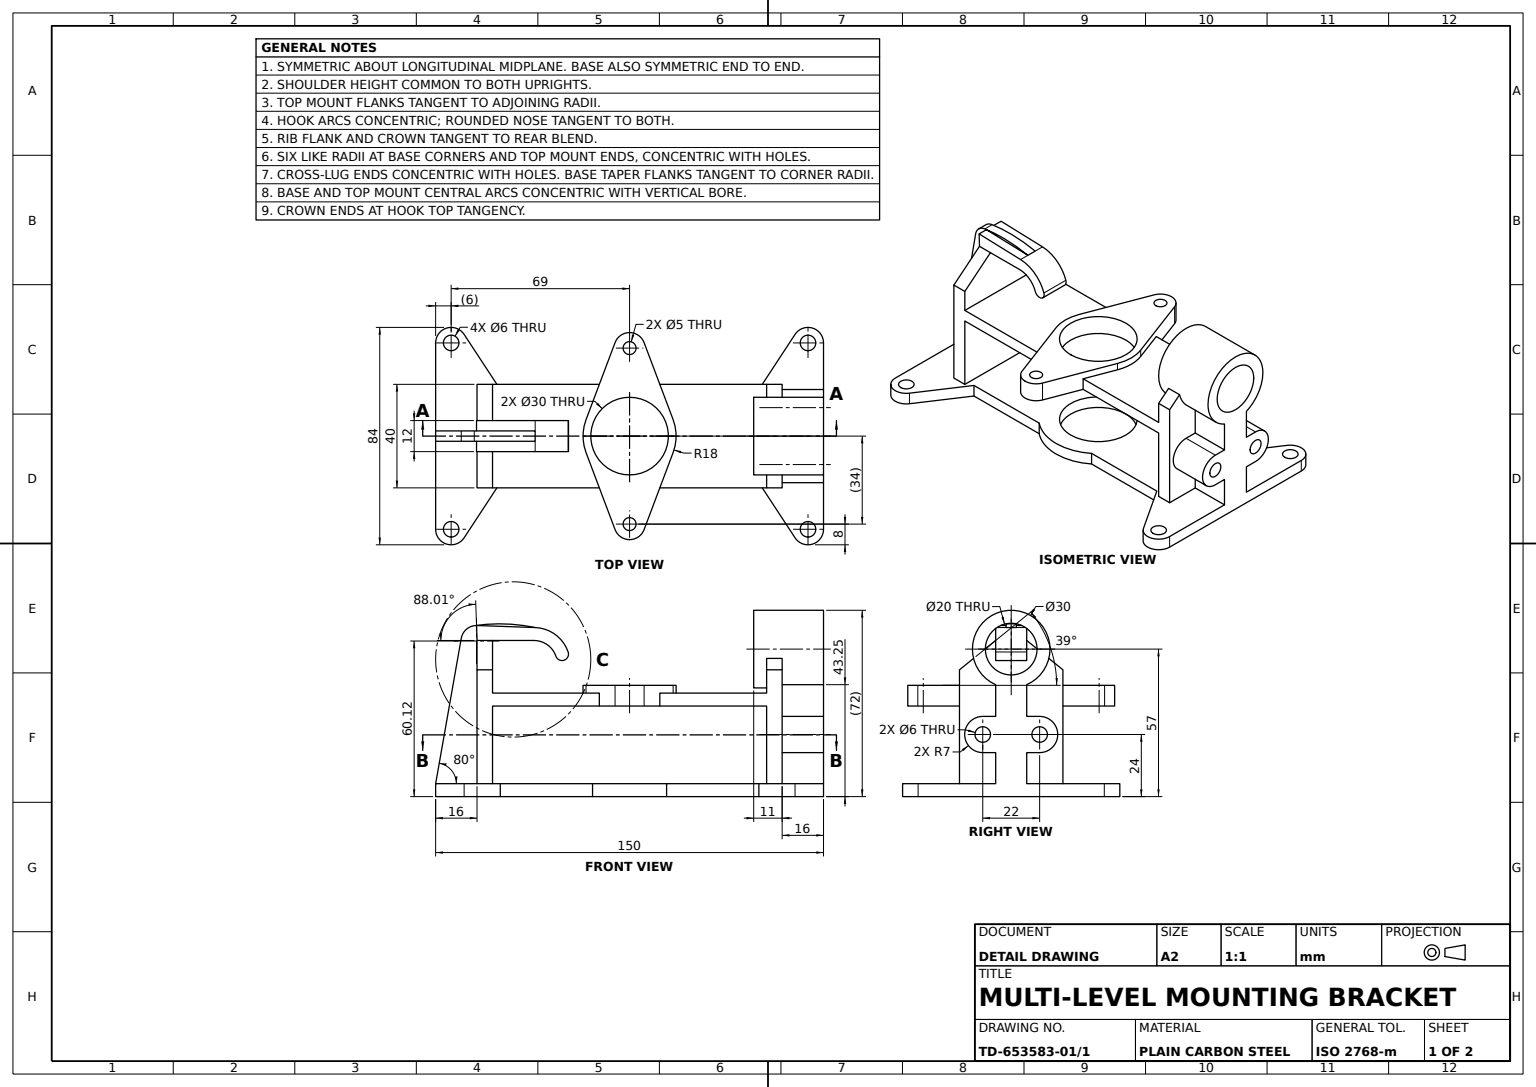
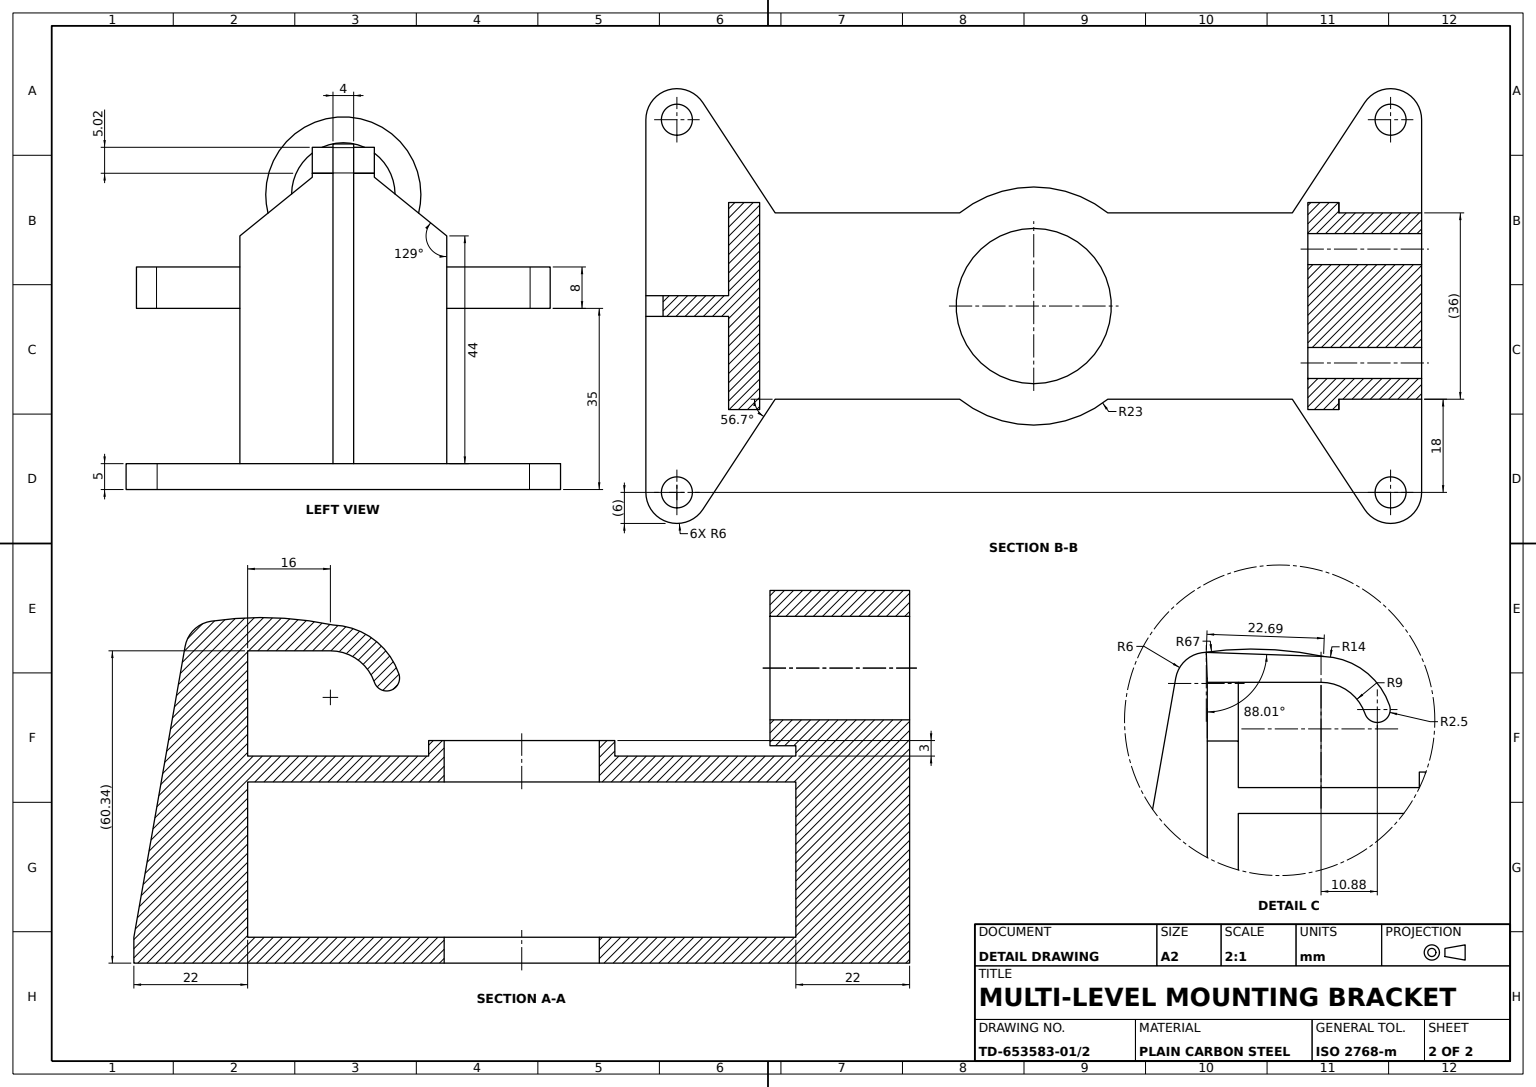
solid
v1 (-53,49,-20)
v2 (-53,40,-20)
e1 v1 v2 LINE
v3 (-53,53.403279,-14.562404)
e2 v1 v3 LINE
v4 (-53,53.403279,14.562404)
e3 v3 v4 CIRCLE(AX(P(-53,57,0),D(-1,0,0),D(0,0,1)),15)
v5 (-53,49,20)
e4 v5 v4 LINE
v6 (-53,40,20)
e5 v5 v6 LINE
e6 v6 v2 LINE
face PLANE(AX(P(-53,49,-20),D(-1,0,0),D(0,0,1))) rev [-e1 e2 e3 -e4 e5 e6]
v7 (0,43,36.5)
v8 (0,43,31.5)
e7 v7 v8 CIRCLE(AX(P(0,43,34),D(0,1,0),D(0,0,1)),2.5)
v9 (0,35,31.5)
e8 v8 v9 LINE
v10 (0,35,36.5)
e9 v10 v9 CIRCLE(AX(P(0,35,34),D(0,1,0),D(0,0,1)),2.5)
e10 v7 v10 LINE
face CYL(AX(P(0,43,34),D(0,-1,0),D(0,0,-1)),2.5) rev [e7 e8 -e9 -e10]
v11 (69,0,33)
v12 (69,0,39)
e11 v11 v12 CIRCLE(AX(P(69,0,36),D(0,1,0),D(0,0,1)),3)
v13 (69,5,33)
e12 v13 v11 LINE
v14 (69,5,39)
e13 v13 v14 CIRCLE(AX(P(69,5,36),D(0,1,0),D(0,0,1)),3)
e14 v14 v12 LINE
face CYL(AX(P(69,5,36),D(0,-1,0),D(0,0,-1)),3) rev [-e11 -e12 e13 e14]
v15 (63.984888,0,39.293729)
v16 (75,0,36)
e15 v15 v16 CIRCLE(AX(P(69,0,36),D(0,1,0),D(0,0,1)),6)
v17 (75,5,36)
e16 v17 v16 LINE
v18 (63.984888,5,39.293729)
e17 v18 v17 CIRCLE(AX(P(69,5,36),D(0,1,0),D(0,0,1)),6)
e18 v18 v15 LINE
face CYL(AX(P(69,5,36),D(0,-1,0),D(0,0,-1)),6) [e15 -e16 -e17 e18]
v19 (59.014781,61.103283,-6)
v20 (59,61.102768,-6)
e19 v19 v20 LINE
v21 (59.014781,61.103283,-2)
e20 v21 v19 LINE
v22 (59,61.102768,-2)
e21 v21 v22 LINE
e22 v20 v22 LINE
face PLANE(AX(P(-2.052934,58.977594,6),D(0.03478765,-0.999394727,0),D(0.999394727,0.03478765,0))) [-e19 -e20 e21 -e22]
v23 (-75,5,-6)
v24 (-75,17,-6)
e23 v23 v24 LINE
v25 (-59,17,-6)
e24 v24 v25 LINE
v26 (-59,5,-6)
e25 v25 v26 LINE
e26 v23 v26 LINE
face PLANE(AX(P(-153,43.252273,-6),D(0,0,1),D(1,0,0))) rev [e23 e24 e25 -e26]
v27 (-5.613873,35,36.117647)
v28 (5.613873,35,36.117647)
e27 v27 v28 CIRCLE(AX(P(0,35,34),D(0,1,0),D(0,0,1)),6)
v29 (5.613873,43,36.117647)
e28 v29 v28 LINE
v30 (-5.613873,43,36.117647)
e29 v30 v29 CIRCLE(AX(P(0,43,34),D(0,1,0),D(0,0,1)),6)
e30 v30 v27 LINE
face CYL(AX(P(0,43,34),D(0,-1,0),D(0,0,-1)),6) [e27 -e28 -e29 e30]
v31 (11.69372,35,-20)
v32 (5.613873,35,-36.117647)
e31 v31 v32 LINE
v33 (53,35,-20)
e32 v31 v33 LINE
v34 (53,35,20)
e33 v33 v34 LINE
v35 (11.69372,35,20)
e34 v35 v34 LINE
e35 v35 v28 LINE
v36 (-11.69372,35,20)
e36 v36 v27 LINE
v37 (-53,35,20)
e37 v37 v36 LINE
v38 (-53,35,-20)
e38 v37 v38 LINE
v39 (-11.69372,35,-20)
e39 v38 v39 LINE
v40 (-5.613873,35,-36.117647)
e40 v39 v40 LINE
v41 (0,35,-40)
e41 v41 v40 CIRCLE(AX(P(0,35,-34),D(0,1,0),D(0,0,1)),6)
e42 v32 v41 CIRCLE(AX(P(0,35,-34),D(0,1,0),D(0,0,1)),6)
e43 v9 v10 CIRCLE(AX(P(0,35,34),D(0,1,0),D(0,0,1)),2.5)
v42 (0,35,15)
v43 (0,35,-15)
e44 v42 v43 CIRCLE(AX(P(0,35,0),D(0,1,0),D(0,0,1)),15)
e45 v43 v42 CIRCLE(AX(P(0,35,0),D(0,1,0),D(0,0,1)),15)
v44 (0,35,-31.5)
v45 (0,35,-36.5)
e46 v44 v45 CIRCLE(AX(P(0,35,-34),D(0,1,0),D(0,0,1)),2.5)
e47 v45 v44 CIRCLE(AX(P(0,35,-34),D(0,1,0),D(0,0,1)),2.5)
face PLANE(AX(P(0,35,0),D(0,1,0),D(0,0,1))) rev [-e31 e32 e33 -e34 e35 -e27 -e36 -e37 e38 e39 e40 -e41 -e42] [e9 e43] [e44 e45] [e46 e47]
v46 (50,5,18)
e48 v46 v18 LINE
v47 (50,0,18)
e49 v46 v47 LINE
e50 v47 v15 LINE
face PLANE(AX(P(63.984888,5,39.293729),D(0.835851987,0,-0.548954875),D(-0.548954875,0,-0.835851987))) rev [-e18 -e48 e49 e50]
v48 (-11.69372,40,20)
e51 v6 v48 LINE
v49 (-16.841619,40,6.352941)
e52 v48 v49 LINE
v50 (-16.841619,40,-6.352941)
e53 v49 v50 CIRCLE(AX(P(0,40,0),D(0,-1,0),D(0,0,1)),18)
v51 (-11.69372,40,-20)
e54 v51 v50 LINE
e55 v2 v51 LINE
face PLANE(AX(P(0,40,0),D(0,1,0),D(0,0,1))) [e51 e52 e53 -e54 -e55 -e6]
v52 (11.69372,40,20)
v53 (53,40,20)
e56 v52 v53 LINE
e57 v52 v35 LINE
v54 (53,5,20)
e58 v34 v54 LINE
v55 (59,5,20)
e59 v54 v55 LINE
v56 (59,49,20)
e60 v56 v55 LINE
v57 (53,49,20)
e61 v57 v56 LINE
e62 v57 v53 LINE
face PLANE(AX(P(-59,49,20),D(0,0,-1),D(-1,0,0))) rev [-e56 e57 e34 e58 e59 -e60 -e61 e62]
v58 (-75,57,10)
v59 (-75,57,-10)
e63 v58 v59 CIRCLE(AX(P(-75,57,0),D(1,0,0),D(0,0,-1)),10)
v60 (-48,57,10)
e64 v60 v58 LINE
v61 (-48,57,-10)
e65 v61 v60 CIRCLE(AX(P(-48,57,0),D(-1,0,0),D(0,0,1)),10)
e66 v61 v59 LINE
face CYL(AX(P(-53,57,0),D(-1,0,0),D(0,0,1)),10) rev [-e63 -e64 -e65 e66]
v62 (16.841619,43,6.352941)
v63 (16.841619,40,6.352941)
e67 v62 v63 LINE
v64 (16.841619,40,-6.352941)
e68 v64 v63 CIRCLE(AX(P(0,40,0),D(0,-1,0),D(0,0,1)),18)
v65 (16.841619,43,-6.352941)
e69 v65 v64 LINE
e70 v62 v65 CIRCLE(AX(P(0,43,0),D(0,1,0),D(0,0,1)),18)
face CYL(AX(P(0,43,0),D(0,-1,0),D(0,0,-1)),18) [e67 -e68 -e69 -e70]
v66 (0,43,15)
v67 (0,43,-15)
e71 v66 v67 CIRCLE(AX(P(0,43,0),D(0,1,0),D(0,0,1)),15)
e72 v67 v43 LINE
e73 v66 v42 LINE
face CYL(AX(P(0,40,0),D(0,-1,0),D(0,0,-1)),15) rev [e71 e72 -e44 -e73]
v68 (59.014781,61.103283,6)
v69 (59.014781,61.103283,2)
e74 v68 v69 LINE
v70 (59,61.102768,6)
e75 v68 v70 LINE
v71 (59,61.102768,2)
e76 v71 v70 LINE
e77 v69 v71 LINE
face PLANE(AX(P(-2.052934,58.977594,6),D(0.03478765,-0.999394727,0),D(0.999394727,0.03478765,0))) [-e74 e75 -e76 -e77]
v72 (14.317821,0,18)
e78 v72 v47 LINE
v73 (14.317821,5,18)
e79 v73 v46 LINE
e80 v73 v72 LINE
face PLANE(AX(P(14.317821,5,18),D(0,0,-1),D(-1,0,0))) rev [e78 -e49 -e79 e80]
v74 (-75,5,36)
v75 (-75,0,36)
e81 v74 v75 LINE
v76 (-63.984888,0,39.293729)
e82 v75 v76 CIRCLE(AX(P(-69,0,36),D(0,1,0),D(0,0,1)),6)
v77 (-63.984888,5,39.293729)
e83 v77 v76 LINE
e84 v74 v77 CIRCLE(AX(P(-69,5,36),D(0,1,0),D(0,0,1)),6)
face CYL(AX(P(-69,5,36),D(0,-1,0),D(0,0,-1)),6) [e81 e82 -e83 -e84]
v78 (69,5,-42)
v79 (63.984888,5,-39.293729)
e85 v78 v79 CIRCLE(AX(P(69,5,-36),D(0,1,0),D(0,0,1)),6)
v80 (69,0,-42)
e86 v78 v80 LINE
v81 (63.984888,0,-39.293729)
e87 v80 v81 CIRCLE(AX(P(69,0,-36),D(0,1,0),D(0,0,1)),6)
e88 v79 v81 LINE
face CYL(AX(P(69,5,-36),D(0,-1,0),D(0,0,-1)),6) [-e85 e86 e87 -e88]
v82 (0,43,-36.5)
e89 v82 v45 LINE
v83 (0,43,-31.5)
e90 v82 v83 CIRCLE(AX(P(0,43,-34),D(0,1,0),D(0,0,1)),2.5)
e91 v83 v44 LINE
face CYL(AX(P(0,43,-34),D(0,-1,0),D(0,0,-1)),2.5) rev [-e89 e90 e91 -e47]
v84 (23.624307,55.074528,6)
v85 (28.488588,54.262017,6)
e92 v84 v85 CIRCLE(AX(P(26.124307,55.074528,6),D(0,0,1),D(1,0,0)),2.5)
v86 (23.624307,55.074528,-6)
e93 v84 v86 LINE
v87 (28.488588,54.262017,-6)
e94 v86 v87 CIRCLE(AX(P(26.124307,55.074528,-6),D(0,0,1),D(1,0,0)),2.5)
e95 v85 v87 LINE
face CYL(AX(P(26.124307,55.074528,6),D(0,0,-1),D(-1,0,0)),2.5) [-e92 e93 e94 -e95]
v88 (36.512973,65.328503,-6)
v89 (23.760025,55.887039,-6)
e96 v88 v89 CIRCLE(AX(P(37,51.336976,-6),D(0,0,1),D(1,0,0)),14)
v90 (23.760025,55.887039,6)
e97 v90 v89 LINE
v91 (36.512973,65.328503,6)
e98 v91 v90 CIRCLE(AX(P(37,51.336976,6),D(0,0,1),D(1,0,0)),14)
v92 (36.512973,65.328503,2)
e99 v91 v92 LINE
v93 (36.512973,65.328503,-2)
e100 v92 v93 LINE
e101 v93 v88 LINE
face CYL(AX(P(37,51.336976,6),D(0,0,-1),D(-1,0,0)),14) [e96 -e97 -e98 e99 e100 e101]
v94 (75,0,-36)
e102 v94 v80 CIRCLE(AX(P(69,0,-36),D(0,1,0),D(0,0,1)),6)
v95 (75,5,-36)
e103 v95 v78 CIRCLE(AX(P(69,5,-36),D(0,1,0),D(0,0,1)),6)
e104 v95 v94 LINE
face CYL(AX(P(69,5,-36),D(0,-1,0),D(0,0,-1)),6) [e102 -e86 -e103 e104]
e105 v52 v63 LINE
e106 v62 v29 LINE
face PLANE(AX(P(16.841619,43,6.352941),D(0.935645513,0,0.352941176),D(0.352941176,0,-0.935645513))) [e105 -e67 e106 e28 -e35 -e57]
v96 (59.188682,66.117815,-6)
e107 v88 v96 LINE
v97 (59.188682,66.117815,-2)
e108 v93 v97 LINE
e109 v97 v96 LINE
face PLANE(AX(P(-2.227062,63.980012,6),D(-0.03478765,0.999394727,0),D(-0.999394727,-0.03478765,0))) [-e107 -e101 e108 e109]
v98 (75,5,2)
v99 (75,5,-2)
e110 v98 v99 LINE
e111 v17 v98 LINE
e112 v16 v94 LINE
e113 v99 v95 LINE
face PLANE(AX(P(75,5,-36),D(-1,0,0),D(0,0,1))) rev [-e110 -e111 e16 e112 -e104 -e113]
v100 (-50,0,18)
e114 v76 v100 LINE
v101 (-50,5,18)
e115 v101 v100 LINE
e116 v77 v101 LINE
face PLANE(AX(P(-63.984888,5,39.293729),D(-0.835851987,0,-0.548954875),D(-0.548954875,0,0.835851987))) rev [e83 e114 -e115 -e116]
e117 v83 v82 CIRCLE(AX(P(0,43,-34),D(0,1,0),D(0,0,1)),2.5)
face CYL(AX(P(0,43,-34),D(0,-1,0),D(0,0,-1)),2.5) rev [-e91 e117 e89 -e46]
v102 (69,0,-33)
v103 (69,0,-39)
e118 v102 v103 CIRCLE(AX(P(69,0,-36),D(0,1,0),D(0,0,1)),3)
e119 v103 v102 CIRCLE(AX(P(69,0,-36),D(0,1,0),D(0,0,1)),3)
v104 (-50,0,-18)
v105 (-63.984888,0,-39.293729)
e120 v104 v105 LINE
v106 (-14.317821,0,-18)
e121 v106 v104 LINE
v107 (0,0,-23)
e122 v107 v106 CIRCLE(AX(P(0,0,0),D(0,1,0),D(0,0,1)),23)
v108 (14.317821,0,-18)
e123 v108 v107 CIRCLE(AX(P(0,0,0),D(0,1,0),D(0,0,1)),23)
v109 (50,0,-18)
e124 v109 v108 LINE
e125 v81 v109 LINE
v110 (-14.317821,0,18)
e126 v110 v72 CIRCLE(AX(P(0,0,0),D(0,1,0),D(0,0,1)),23)
e127 v100 v110 LINE
v111 (-75,0,-36)
e128 v111 v75 LINE
v112 (-69,0,-42)
e129 v112 v111 CIRCLE(AX(P(-69,0,-36),D(0,1,0),D(0,0,1)),6)
e130 v105 v112 CIRCLE(AX(P(-69,0,-36),D(0,1,0),D(0,0,1)),6)
v113 (-69,0,-33)
v114 (-69,0,-39)
e131 v113 v114 CIRCLE(AX(P(-69,0,-36),D(0,1,0),D(0,0,1)),3)
e132 v114 v113 CIRCLE(AX(P(-69,0,-36),D(0,1,0),D(0,0,1)),3)
v115 (0,0,-15)
v116 (0,0,15)
e133 v115 v116 CIRCLE(AX(P(0,0,0),D(0,1,0),D(0,0,1)),15)
e134 v116 v115 CIRCLE(AX(P(0,0,0),D(0,1,0),D(0,0,1)),15)
e135 v12 v11 CIRCLE(AX(P(69,0,36),D(0,1,0),D(0,0,1)),3)
v117 (-69,0,33)
v118 (-69,0,39)
e136 v117 v118 CIRCLE(AX(P(-69,0,36),D(0,1,0),D(0,0,1)),3)
e137 v118 v117 CIRCLE(AX(P(-69,0,36),D(0,1,0),D(0,0,1)),3)
face PLANE(AX(P(0,0,0),D(0,1,0),D(0,0,1))) rev [e118 e119] [-e120 -e121 -e122 -e123 -e124 -e125 -e87 -e102 -e112 -e15 -e50 -e78 -e126 -e127 -e114 -e82 -e128 -e129 -e130] [e131 e132] [e133 e134] [e11 e135] [e136 e137]
e138 v90 v84 CIRCLE(AX(P(26.124307,55.074528,6),D(0,0,1),D(1,0,0)),2.5)
e139 v89 v86 CIRCLE(AX(P(26.124307,55.074528,-6),D(0,0,1),D(1,0,0)),2.5)
face CYL(AX(P(26.124307,55.074528,6),D(0,0,-1),D(-1,0,0)),2.5) [-e138 e97 e139 -e93]
e140 v48 v36 LINE
v119 (-16.841619,43,6.352941)
e141 v119 v30 LINE
e142 v119 v49 LINE
face PLANE(AX(P(-16.841619,43,6.352941),D(0.935645513,0,-0.352941176),D(-0.352941176,0,-0.935645513))) rev [-e52 e140 e36 -e30 -e141 e142]
v120 (65.097529,61.159704,-2)
e143 v99 v120 LINE
v121 (65.097529,61.159704,2)
e144 v121 v120 LINE
e145 v98 v121 LINE
face PLANE(AX(P(75,5,2),D(-0.984807753,-0.173648178,0),D(0.173648178,-0.984807753,0))) rev [e110 e143 -e144 -e145]
v122 (-16.841619,43,-6.352941)
e146 v122 v50 LINE
e147 v122 v119 CIRCLE(AX(P(0,43,0),D(0,1,0),D(0,0,1)),18)
face CYL(AX(P(0,43,0),D(0,-1,0),D(0,0,-1)),18) [e146 -e53 -e142 -e147]
v123 (5.613873,43,-36.117647)
v124 (0,43,-40)
e148 v123 v124 CIRCLE(AX(P(0,43,-34),D(0,1,0),D(0,0,1)),6)
e149 v123 v32 LINE
e150 v124 v41 LINE
face CYL(AX(P(0,43,-34),D(0,-1,0),D(0,0,-1)),6) [-e148 e149 e42 -e150]
v125 (-59,5,6)
v126 (-59,17,6)
e151 v125 v126 LINE
v127 (-75,17,6)
e152 v126 v127 LINE
v128 (-75,5,6)
e153 v127 v128 LINE
e154 v125 v128 LINE
face PLANE(AX(P(-153,43.252273,6),D(0,0,-1),D(-1,0,0))) rev [e151 e152 e153 -e154]
v129 (50,5,-18)
e155 v79 v129 LINE
e156 v129 v109 LINE
face PLANE(AX(P(63.984888,5,-39.293729),D(0.835851987,0,0.548954875),D(0.548954875,0,-0.835851987))) rev [-e155 e88 e125 -e156]
e157 v8 v7 CIRCLE(AX(P(0,43,34),D(0,1,0),D(0,0,1)),2.5)
face CYL(AX(P(0,43,34),D(0,-1,0),D(0,0,-1)),2.5) rev [e157 e10 -e43 -e8]
v130 (-5.613873,43,-36.117647)
e158 v122 v130 LINE
e159 v130 v40 LINE
e160 v51 v39 LINE
face PLANE(AX(P(-16.841619,43,-6.352941),D(-0.935645513,0,-0.352941176),D(-0.352941176,0,0.935645513))) [e158 e159 -e40 -e160 e54 -e146]
v131 (-75,31,6)
v132 (-75,31,11)
e161 v131 v132 LINE
v133 (-59,31,11)
e162 v133 v132 LINE
v134 (-59,31,6)
e163 v134 v133 LINE
e164 v134 v131 LINE
face PLANE(AX(P(-20.373584,31,0),D(0,-1,0),D(0,0,-1))) rev [e161 -e162 -e163 e164]
v135 (-59,49,20)
v136 (-59,53.403279,14.562404)
e165 v135 v136 LINE
e166 v135 v5 LINE
e167 v4 v136 LINE
face PLANE(AX(P(-53,39.375312,31.885499),D(0,0.777145961,0.629320391),D(0,-0.629320391,0.777145961))) [-e165 e166 e4 e167]
e168 v96 v19 LINE
e169 v97 v21 LINE
face PLANE(AX(P(56.827402,-1.970749,6),D(0.999399206,-0.034658712,0),D(0.034658712,0.999399206,0))) [e20 -e168 -e109 e169]
v137 (59.188682,66.117815,6)
e170 v137 v68 LINE
e171 v91 v137 LINE
v138 (37,60.336976,6)
e172 v138 v85 CIRCLE(AX(P(37,51.336976,6),D(0,0,1),D(1,0,0)),9)
v139 (53,60.336976,6)
e173 v138 v139 LINE
v140 (59,60.336976,6)
e174 v139 v140 LINE
e175 v140 v70 LINE
face PLANE(AX(P(37,0,6),D(0,0,-1),D(-1,0,0))) rev [-e75 -e170 -e171 e98 e138 e92 -e172 e173 e174 e175]
v141 (53,49,-20)
v142 (53,60.336976,-6)
e176 v141 v142 LINE
v143 (59,60.336976,-6)
e177 v142 v143 LINE
v144 (59,49,-20)
e178 v144 v143 LINE
e179 v144 v141 LINE
face PLANE(AX(P(53,39.375312,-31.885499),D(0,0.777145961,-0.629320391),D(0,0.629320391,0.777145961))) [e176 e177 -e178 e179]
v145 (14.317821,5,-18)
e180 v145 v108 LINE
e181 v129 v145 LINE
face PLANE(AX(P(14.317821,5,-18),D(0,0,1),D(1,0,0))) rev [-e180 -e181 e156 e124]
e182 v67 v66 CIRCLE(AX(P(0,43,0),D(0,1,0),D(0,0,1)),15)
e183 v65 v123 LINE
e184 v124 v130 CIRCLE(AX(P(0,43,-34),D(0,1,0),D(0,0,1)),6)
face PLANE(AX(P(0,43,0),D(0,1,0),D(0,0,1))) [-e71 -e182] [-e106 e70 e183 e148 e184 -e158 e147 e141 e29] [-e90 -e117] [-e7 -e157]
v146 (-59,17,11)
v147 (-75,17,11)
e185 v146 v147 LINE
v148 (-59,24,18)
e186 v146 v148 CIRCLE(AX(P(-59,24,11),D(-1,0,0),D(0,0,-1)),7)
v149 (-75,24,18)
e187 v148 v149 LINE
e188 v147 v149 CIRCLE(AX(P(-75,24,11),D(-1,0,0),D(0,0,1)),7)
face CYL(AX(P(-20.373584,24,11),D(-1,0,0),D(0,0,1)),7) [-e185 e186 e187 -e188]
v150 (60.061182,66.054038,2)
v151 (60.061182,66.054038,-2)
e189 v150 v151 LINE
e190 v121 v150 CIRCLE(AX(P(59.188682,60.117815,2),D(0,0,1),D(-1,0,0)),6)
e191 v120 v151 CIRCLE(AX(P(59.188682,60.117815,-2),D(0,0,1),D(-1,0,0)),6)
face CYL(AX(P(59.188682,60.117815,2),D(0,0,-1),D(-1,0,0)),6) [-e189 -e190 e144 e191]
e192 v14 v13 CIRCLE(AX(P(69,5,36),D(0,1,0),D(0,0,1)),3)
face CYL(AX(P(69,5,36),D(0,-1,0),D(0,0,-1)),3) rev [-e135 -e14 e192 e12]
v152 (-69,5,33)
e193 v152 v117 LINE
v153 (-69,5,39)
e194 v153 v118 LINE
e195 v153 v152 CIRCLE(AX(P(-69,5,36),D(0,1,0),D(0,0,1)),3)
face CYL(AX(P(-69,5,36),D(0,-1,0),D(0,0,-1)),3) rev [e193 -e137 -e194 e195]
v154 (-50,5,-18)
e196 v154 v104 LINE
v155 (-63.984888,5,-39.293729)
e197 v155 v105 LINE
e198 v154 v155 LINE
face PLANE(AX(P(-50,5,-18),D(-0.835851987,0,0.548954875),D(0.548954875,0,0.835851987))) rev [e196 e120 -e197 -e198]
v156 (-69,5,-39)
e199 v156 v114 LINE
v157 (-69,5,-33)
e200 v157 v113 LINE
e201 v157 v156 CIRCLE(AX(P(-69,5,-36),D(0,1,0),D(0,0,1)),3)
face CYL(AX(P(-69,5,-36),D(0,-1,0),D(0,0,-1)),3) rev [e199 -e131 -e200 e201]
v158 (59,5,-2)
e202 v22 v158 LINE
v159 (59,5,-20)
e203 v158 v159 LINE
e204 v144 v159 LINE
e205 v143 v20 LINE
face PLANE(AX(P(59,49,-20),D(-1,0,0),D(0,0,1))) rev [e22 e202 e203 -e204 e178 e205]
e206 v139 v142 LINE
v160 (37,60.336976,-6)
e207 v138 v160 LINE
e208 v160 v142 LINE
face PLANE(AX(P(37,60.336976,0),D(0,-1,0),D(0,0,-1))) [-e206 -e173 e207 e208]
v161 (69,5,-39)
v162 (69,5,-33)
e209 v161 v162 CIRCLE(AX(P(69,5,-36),D(0,1,0),D(0,0,1)),3)
e210 v162 v161 CIRCLE(AX(P(69,5,-36),D(0,1,0),D(0,0,1)),3)
e211 v156 v157 CIRCLE(AX(P(-69,5,-36),D(0,1,0),D(0,0,1)),3)
e212 v152 v153 CIRCLE(AX(P(-69,5,36),D(0,1,0),D(0,0,1)),3)
v163 (0,5,-15)
v164 (0,5,15)
e213 v163 v164 CIRCLE(AX(P(0,5,0),D(0,1,0),D(0,0,1)),15)
e214 v164 v163 CIRCLE(AX(P(0,5,0),D(0,1,0),D(0,0,1)),15)
e215 v158 v99 LINE
v165 (0,5,-23)
e216 v145 v165 CIRCLE(AX(P(0,5,0),D(0,1,0),D(0,0,1)),23)
v166 (-14.317821,5,-18)
e217 v165 v166 CIRCLE(AX(P(0,5,0),D(0,1,0),D(0,0,1)),23)
e218 v166 v154 LINE
v167 (-69,5,-42)
e219 v155 v167 CIRCLE(AX(P(-69,5,-36),D(0,1,0),D(0,0,1)),6)
v168 (-75,5,-36)
e220 v167 v168 CIRCLE(AX(P(-69,5,-36),D(0,1,0),D(0,0,1)),6)
e221 v168 v23 LINE
v169 (-59,5,-20)
e222 v169 v26 LINE
v170 (-53,5,-20)
e223 v170 v169 LINE
v171 (-53,5,20)
e224 v171 v170 LINE
v172 (-59,5,20)
e225 v172 v171 LINE
e226 v125 v172 LINE
e227 v128 v74 LINE
v173 (-14.317821,5,18)
e228 v101 v173 LINE
e229 v173 v73 CIRCLE(AX(P(0,5,0),D(0,1,0),D(0,0,1)),23)
v174 (59,5,2)
e230 v174 v98 LINE
e231 v55 v174 LINE
v175 (53,5,-20)
e232 v175 v54 LINE
e233 v159 v175 LINE
face PLANE(AX(P(0,5,0),D(0,1,0),D(0,0,1))) [-e209 -e210] [-e211 -e201] [-e13 -e192] [-e195 -e212] [-e213 -e214] [-e203 e215 e113 e103 e85 e155 e181 e216 e217 e218 e198 e219 e220 e221 e26 -e222 -e223 -e224 -e225 -e226 e154 e227 e84 e116 e228 e229 e79 e48 e17 e111 -e230 -e231 -e59 -e232 -e233]
v176 (-59,43.252273,6)
e234 v176 v136 CIRCLE(AX(P(-59,57,0),D(-1,0,0),D(0,0,1)),15)
e235 v134 v176 LINE
e236 v148 v133 CIRCLE(AX(P(-59,24,11),D(-1,0,0),D(0,0,-1)),7)
e237 v126 v146 LINE
e238 v135 v172 LINE
face PLANE(AX(P(-59,49,-20),D(1,0,0),D(0,0,-1))) rev [e165 -e234 -e235 e163 -e236 -e186 -e237 -e151 e226 -e238]
v177 (-59,53.403279,-14.562404)
e239 v3 v177 LINE
v178 (-59,43.252273,-6)
e240 v177 v178 CIRCLE(AX(P(-59,57,0),D(-1,0,0),D(0,0,1)),15)
v179 (-75,43.252273,-6)
e241 v179 v178 LINE
v180 (-75,57,-15)
e242 v179 v180 CIRCLE(AX(P(-75,57,0),D(1,0,0),D(0,0,-1)),15)
v181 (-48,57,-15)
e243 v181 v180 LINE
v182 (-48,57,15)
e244 v181 v182 CIRCLE(AX(P(-48,57,0),D(-1,0,0),D(0,0,1)),15)
v183 (-75,57,15)
e245 v182 v183 LINE
v184 (-75,43.252273,6)
e246 v183 v184 CIRCLE(AX(P(-75,57,0),D(1,0,0),D(0,0,-1)),15)
e247 v184 v176 LINE
face CYL(AX(P(-53,57,0),D(-1,0,0),D(0,0,1)),15) [-e3 e239 e240 -e241 e242 -e243 e244 e245 e246 e247 e234 -e167]
e248 v167 v112 LINE
face CYL(AX(P(-69,5,-36),D(0,-1,0),D(0,0,-1)),6) [-e219 e197 e130 -e248]
v185 (-59,31,-11)
v186 (-59,31,-6)
e249 v185 v186 LINE
e250 v178 v186 LINE
v187 (-59,49,-20)
e251 v187 v177 LINE
e252 v187 v169 LINE
v188 (-59,17,-11)
e253 v188 v25 LINE
e254 v185 v188 CIRCLE(AX(P(-59,24,-11),D(-1,0,0),D(0,0,-1)),7)
face PLANE(AX(P(-59,49,-20),D(1,0,0),D(0,0,-1))) rev [e249 -e250 -e240 -e251 e252 e222 -e25 -e253 -e254]
v189 (-75,24,14)
v190 (-75,24,8)
e255 v189 v190 CIRCLE(AX(P(-75,24,11),D(-1,0,0),D(0,0,1)),3)
v191 (-53,24,8)
e256 v191 v190 LINE
v192 (-53,24,14)
e257 v192 v191 CIRCLE(AX(P(-53,24,11),D(-1,0,0),D(0,0,1)),3)
e258 v192 v189 LINE
face CYL(AX(P(-20.373584,24,11),D(-1,0,0),D(0,0,1)),3) rev [e255 -e256 -e257 e258]
v193 (-53,24,-14)
v194 (-53,24,-8)
e259 v193 v194 CIRCLE(AX(P(-53,24,-11),D(-1,0,0),D(0,0,1)),3)
v195 (-75,24,-14)
e260 v193 v195 LINE
v196 (-75,24,-8)
e261 v195 v196 CIRCLE(AX(P(-75,24,-11),D(-1,0,0),D(0,0,1)),3)
e262 v194 v196 LINE
face CYL(AX(P(-20.373584,24,-11),D(-1,0,0),D(0,0,1)),3) rev [-e259 e260 e261 -e262]
e263 v162 v102 LINE
e264 v161 v103 LINE
face CYL(AX(P(69,5,-36),D(0,-1,0),D(0,0,-1)),3) rev [e263 -e119 -e264 e209]
face CYL(AX(P(69,5,-36),D(0,-1,0),D(0,0,-1)),3) rev [-e263 e210 e264 -e118]
v197 (59.188682,66.117815,2)
e265 v197 v69 LINE
e266 v137 v197 LINE
face PLANE(AX(P(56.827402,-1.970749,6),D(0.999399206,-0.034658712,0),D(0.034658712,0.999399206,0))) [-e265 -e266 e170 e74]
e267 v57 v139 LINE
v198 (53,40,-20)
e268 v141 v198 LINE
e269 v198 v53 LINE
face PLANE(AX(P(53,49,-20),D(1,0,0),D(0,0,-1))) rev [e267 e206 -e176 e268 e269 -e62]
face CYL(AX(P(-69,5,-36),D(0,-1,0),D(0,0,-1)),3) rev [e211 e200 -e132 -e199]
v199 (-75,31,-6)
e270 v199 v186 LINE
v200 (-75,31,-11)
e271 v185 v200 LINE
e272 v200 v199 LINE
face PLANE(AX(P(-20.373584,31,0),D(0,-1,0),D(0,0,-1))) rev [e270 -e249 e271 e272]
e273 v182 v181 CIRCLE(AX(P(-48,57,0),D(-1,0,0),D(0,0,1)),15)
e274 v180 v183 CIRCLE(AX(P(-75,57,0),D(1,0,0),D(0,0,-1)),15)
face CYL(AX(P(-53,57,0),D(-1,0,0),D(0,0,1)),15) [e273 e243 e274 -e245]
v201 (11.69372,40,-20)
e275 v201 v198 LINE
e276 v201 v64 LINE
face PLANE(AX(P(0,40,0),D(0,1,0),D(0,0,1))) [e56 -e269 -e275 e276 e68 -e105]
e277 v92 v197 LINE
face PLANE(AX(P(-2.227062,63.980012,6),D(-0.03478765,0.999394727,0),D(-0.999394727,-0.03478765,0))) [-e99 e171 e266 -e277]
v202 (-75,17,-11)
e278 v200 v202 CIRCLE(AX(P(-75,24,-11),D(-1,0,0),D(0,0,1)),7)
e279 v188 v202 LINE
face CYL(AX(P(-20.373584,24,-11),D(-1,0,0),D(0,0,1)),7) [-e278 -e271 e254 e279]
face CYL(AX(P(0,43,-34),D(0,-1,0),D(0,0,-1)),6) [e150 e41 -e159 -e184]
e280 v38 v170 LINE
e281 v37 v171 LINE
e282 v194 v193 CIRCLE(AX(P(-53,24,-11),D(-1,0,0),D(0,0,1)),3)
e283 v191 v192 CIRCLE(AX(P(-53,24,11),D(-1,0,0),D(0,0,1)),3)
face PLANE(AX(P(-53,49,-20),D(-1,0,0),D(0,0,1))) rev [-e280 -e38 e281 e224] [e282 e259] [e283 e257]
e284 v59 v58 CIRCLE(AX(P(-75,57,0),D(1,0,0),D(0,0,-1)),10)
e285 v168 v111 LINE
e286 v127 v147 LINE
e287 v149 v132 CIRCLE(AX(P(-75,24,11),D(-1,0,0),D(0,0,1)),7)
e288 v184 v131 LINE
e289 v199 v179 LINE
e290 v202 v24 LINE
e291 v190 v189 CIRCLE(AX(P(-75,24,11),D(-1,0,0),D(0,0,1)),3)
e292 v196 v195 CIRCLE(AX(P(-75,24,-11),D(-1,0,0),D(0,0,1)),3)
face PLANE(AX(P(-75,5,-36),D(1,0,0),D(0,0,-1))) rev [e63 e284] [e285 e128 -e81 -e227 -e153 e286 e188 e287 -e161 -e288 -e246 -e274 -e242 -e289 -e272 e278 e290 -e23 -e221] [-e291 -e255] [-e292 -e261]
e293 v165 v107 LINE
face CYL(AX(P(0,5,0),D(0,-1,0),D(0,0,-1)),23) [-e293 -e216 e180 e123]
face CYL(AX(P(-69,5,-36),D(0,-1,0),D(0,0,-1)),6) [e248 e129 -e285 -e220]
e294 v71 v174 LINE
e295 v56 v140 LINE
face PLANE(AX(P(59,49,-20),D(-1,0,0),D(0,0,1))) rev [e60 e231 -e294 e76 -e175 -e295]
e296 v33 v175 LINE
face PLANE(AX(P(53,49,-20),D(1,0,0),D(0,0,-1))) rev [e232 -e58 -e33 e296]
e297 v166 v106 LINE
face CYL(AX(P(0,5,0),D(0,-1,0),D(0,0,-1)),23) [-e297 -e217 e293 e122]
e298 v201 v31 LINE
face PLANE(AX(P(16.841619,43,-6.352941),D(-0.935645513,0,0.352941176),D(0.352941176,0,0.935645513))) rev [-e183 e69 -e276 e298 e31 -e149]
e299 v60 v61 CIRCLE(AX(P(-48,57,0),D(-1,0,0),D(0,0,1)),10)
face CYL(AX(P(-53,57,0),D(-1,0,0),D(0,0,1)),10) rev [e64 -e284 -e66 -e299]
face CYL(AX(P(0,40,0),D(0,-1,0),D(0,0,-1)),15) rev [-e72 e182 e73 -e45]
e300 v160 v87 CIRCLE(AX(P(37,51.336976,-6),D(0,0,1),D(1,0,0)),9)
face CYL(AX(P(37,51.336976,6),D(0,0,-1),D(-1,0,0)),9) rev [-e207 e172 e95 -e300]
e301 v92 v150 CIRCLE(AX(P(50.318271,-0.233786,2),D(0,0,-1),D(1,0,0)),67)
face PLANE(AX(P(59.188682,60.117815,2),D(0,0,-1),D(-1,0,0))) rev [e145 e190 -e301 e277 e265 e77 e294 e230]
face PLANE(AX(P(-153,43.252273,6),D(0,0,-1),D(-1,0,0))) rev [-e164 e235 -e247 e288]
face PLANE(AX(P(-20.373584,17,0),D(0,-1,0),D(0,0,-1))) [-e152 e237 e185 -e286]
face PLANE(AX(P(-50,5,-18),D(0,0,1),D(1,0,0))) rev [-e218 e297 e121 -e196]
e302 v93 v151 CIRCLE(AX(P(50.318271,-0.233786,-2),D(0,0,-1),D(1,0,0)),67)
face PLANE(AX(P(59.188682,60.117815,-2),D(0,0,-1),D(-1,0,0))) [-e108 e302 -e191 -e143 -e215 -e202 -e21 -e169]
face CYL(AX(P(50.318271,-0.233786,2),D(0,0,-1),D(-1,0,0)),67) [-e100 e301 e189 -e302]
face CYL(AX(P(-20.373584,24,11),D(-1,0,0),D(0,0,1)),3) rev [-e258 -e283 e256 e291]
e303 v1 v187 LINE
face PLANE(AX(P(-59,49,-20),D(0,0,1),D(1,0,0))) rev [e160 -e39 e280 e223 -e252 -e303 e1 e55]
face CYL(AX(P(-20.373584,24,-11),D(-1,0,0),D(0,0,1)),3) rev [e262 e292 -e260 -e282]
face PLANE(AX(P(37,0,-6),D(0,0,-1),D(-1,0,0))) [e19 -e205 -e177 -e208 e300 -e94 -e139 -e96 e107 e168]
face PLANE(AX(P(53,39.375312,31.885499),D(0,-0.777145961,-0.629320391),D(0,0.629320391,-0.777145961))) rev [e295 -e174 -e267 e61]
e304 v163 v115 LINE
e305 v164 v116 LINE
face CYL(AX(P(0,5,0),D(0,-1,0),D(0,0,-1)),15) rev [-e133 -e304 e213 e305]
face CYL(AX(P(-20.373584,24,11),D(-1,0,0),D(0,0,1)),7) [e236 e162 -e287 -e187]
face CYL(AX(P(-69,5,36),D(0,-1,0),D(0,0,-1)),3) rev [-e136 -e193 e212 e194]
e306 v173 v110 LINE
face PLANE(AX(P(-50,5,18),D(0,0,-1),D(-1,0,0))) rev [-e306 -e228 e115 e127]
face PLANE(AX(P(-59,49,20),D(0,0,-1),D(-1,0,0))) rev [-e166 e238 e225 -e281 e37 -e140 -e51 -e5]
face PLANE(AX(P(-20.373584,17,0),D(0,-1,0),D(0,0,-1))) [-e24 -e290 -e279 e253]
face PLANE(AX(P(-153,43.252273,-6),D(0,0,1),D(1,0,0))) rev [-e270 e289 e241 e250]
face CYL(AX(P(0,5,0),D(0,-1,0),D(0,0,-1)),23) [-e229 e306 e126 -e80]
face PLANE(AX(P(-59,49,-20),D(0,0,1),D(1,0,0))) rev [e275 -e268 -e179 e204 e233 -e296 -e32 -e298]
face PLANE(AX(P(-53,39.375312,-31.885499),D(0,-0.777145961,0.629320391),D(0,-0.629320391,-0.777145961))) rev [-e2 e303 e251 -e239]
face CYL(AX(P(0,5,0),D(0,-1,0),D(0,0,-1)),15) rev [e214 e304 -e134 -e305]
face PLANE(AX(P(-48,0,0),D(-1,0,0),D(0,0,1))) rev [-e273 -e244] [e299 e65]
